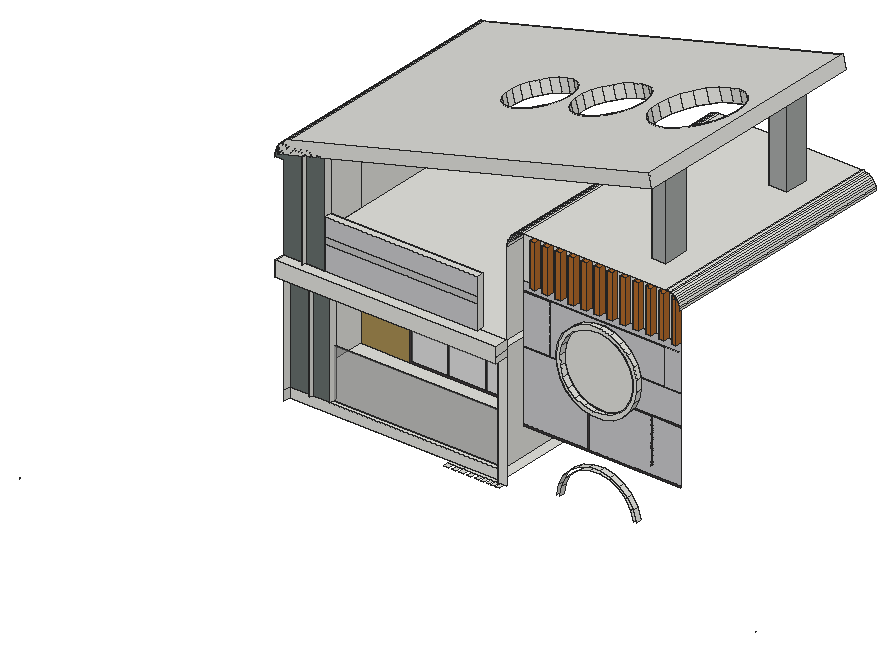
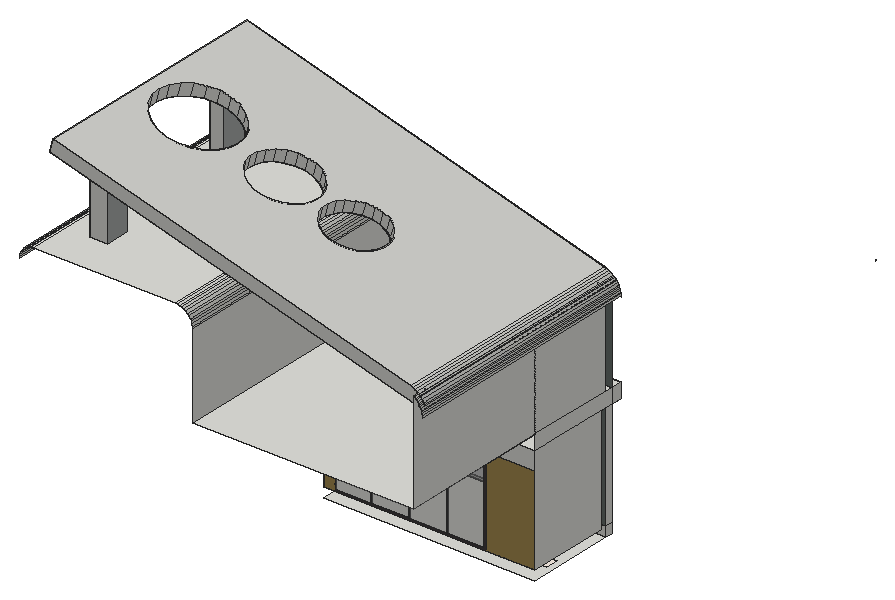
# SketchUp Ruby script. Lengths in inches.
U = 1.inch
M = Sketchup.active_model
def pt(a) = Geom::Point3d.new(a.map { |v| v * U })
def face(e, loops, mat)
  f = e.add_face(loops[0].map { |a| pt(a) })
  loops[1..].each { |l| e.add_face(l.map { |a| pt(a) }).erase! }
  f.material = f.back_material = mat if mat
  f
end
# faces: each face lists its corners as indices into pts; further lists are holes
def faces(e, pts, list, mat = nil) = list.each { |f| face(e, (f[0].is_a?(Array) ? f : [f]).map { |l| l.map { |i| pts[i] } }, mat) }
# xy, xz, yz: faces in a plane at the given z, y or x. An outline is a flat list of corners, or four numbers for a rectangle; further outlines are holes
def ring(l) = l.size == 4 ? [[l[0], l[1]], [l[2], l[1]], [l[2], l[3]], [l[0], l[3]]] : l.each_slice(2).to_a
def flat(e, list, mat, &to3) = list.each { |f| face(e, (f[0].is_a?(Array) ? f : [f]).map { |l| ring(l).map { |u, v| to3.(u, v) } }, mat) }
def xy(e, z, list, mat = nil) = flat(e, list, mat) { |x, y| [x, y, z] }
def xz(e, y, list, mat = nil) = flat(e, list, mat) { |x, z| [x, y, z] }
def yz(e, x, list, mat = nil) = flat(e, list, mat) { |y, z| [x, y, z] }
def lines(e, pts, list) = list.each { |a, b| e.add_line(pt(pts[a]), pt(pts[b])) }
# prism: a flat outline (further loops are holes) pulled along v
def prism(e, loops, v, mat = nil)
  f = face(e, loops, mat); d = Geom::Vector3d.new(v.map { |x| x * U })
  f.pushpull(f.normal.samedirection?(d) ? d.length : -d.length)
end
def box(e, o, s, mat = nil) = prism(e, [[o, [o[0] + s[0], o[1], o[2]], [o[0] + s[0], o[1] + s[1], o[2]], [o[0], o[1] + s[1], o[2]]]], [0, 0, s[2]], mat)
def at(x, y, z, deg = 0) = Geom::Transformation.translation(pt([x, y, z])) * Geom::Transformation.rotation(ORIGIN, Z_AXIS, deg.degrees)
def axes(o, x, y, z) = Geom::Transformation.new([*x, 0, *y, 0, *z, 0, *pt(o).to_a, 1])
def part(name) = M.definitions.add(name)
# library, detail: a bought-in or finely detailed component or shape, given as its bounding box
def library(name, o, s) = part(name).tap { |d| box(d.entities, o, s) }
def detail(e, o, s) = box(e.add_group.entities, o, s)
def put(e, d, t, mat = nil) = e.add_instance(d, t).tap { |i| i.material = mat if mat }
def group(e, t, mat = nil) = e.add_group.tap { |g| g.transformation = t; g.material = mat if mat }.entities
root = M.entities
M.materials.add("Polis06_194").color = [79, 50, 36]
M.materials.add("[0009_Linen]").color = [250, 240, 230]
M.materials.add("[0045_Goldenrod]").color = [218, 165, 32]
M.materials.add("[Asphalt New]").color = [67, 60, 62]
M.materials.add("[Brick Rough Tan]").color = [167, 141, 82]
M.materials.add("[Concrete Form 4x8]").color = [167, 170, 168]
M.materials.add("[Metal Corrugated Shiny]").color = [193, 193, 193]
M.materials.add("[Polished Concrete New]").color = [200, 200, 203]
M.materials.add("[Slate]").color = [102, 110, 108]
M.materials.add("[Translucent Glass Gray]").color = [128, 128, 128]
M.materials["[Translucent Glass Gray]"].alpha = 0.5
M.materials.add("[Wood Bamboo]").color = [177, 105, 43]
c1 = library("Vaso decorativo com seixos\#1",[6.14,-4.72,0],[9.45,4.72,3.26])
c2 = part("群组\#3")
xy(c2.entities,0,[[0,0,4.72,1.18],[0,34.25,4.72,35.43]],"Polis06_194")
xy(c2.entities,85.26,[[0,1.18,4.72,34.25]],"Polis06_194")
xy(c2.entities,86.61,[[0,0,4.72,35.43]],"Polis06_194")
xz(c2.entities,0,[[0,0,4.72,86.61]],"Polis06_194")
xz(c2.entities,1.18,[[0,0,2.36,85.26],[2.36,0,4.72,85.26]],"Polis06_194")
xz(c2.entities,34.25,[[0,0,4.72,85.26]],"Polis06_194")
xz(c2.entities,35.43,[[0,0,4.72,86.61]],"Polis06_194")
yz(c2.entities,0,[[0,0,1.18,86.61],[34.25,0,35.43,86.61],[1.18,85.26,34.25,86.61]],"Polis06_194")
yz(c2.entities,2.36,[[1.18,0,34.25,0,34.25,85.21,1.18,85.26]],"Polis06_194")
yz(c2.entities,4.72,[[0,0,1.18,86.61],[34.25,0,35.43,86.61],[1.18,85.26,34.25,86.61]],"Polis06_194")
xy(root,25308.0625,[[41914.25,35829.26,42429.61,36436.82],[42781.34,35829.26,43218.625,36436.82],[43484.85,35829.26,43975.34,36436.82],[44363.15,35829.26,44725.28,36436.82],[45185.32,35829.26,45537.5,36436.82],
  [45797.6,35829.26,46078.9,36436.82],[46362.66,35829.26,46652.53,36436.82],[46862.23,35829.26,47214.9,36436.82],[47390.11,35829.26,47723.54,36436.82],[41914.25,36436.82,47071.94,36851.76],
  [25070.75,36851.76,47071.94,46071.33]])
xy(root,25456.33,[[25598.07,42633.68,26902.95,43938.55]],"[0009_Linen]")
xy(root,26331.5625,[[27255.29,36569.45,27430.61,36851.76],[29282.19,36851.76,47071.94,37215.15],[29282.19,37327.67,47071.94,37327.67,47071.94,46071.33,25070.75,46071.33,25070.75,37578.54,29282.19,37578.54]])
xy(root,31526.6875,[[29282.19,37215.15,47071.94,37327.67]])
xy(root,37403.375,[[25070.75,34935.13,25070.75,36851.76,27255.29,36851.76,27255.29,36569.45,27430.61,36569.45,27430.61,36851.76,29282.19,36851.76,29282.19,37578.54,25070.75,37578.54,25070.75,46071.33,47071.94,46071.33,47071.94,34935.13],[47071.94,34935.13,48032.1875,36436.82],[27255.29,36569.45,27255.29,36851.76,25070.75,36851.76,25070.75,37578.54,29282.19,37578.54,29282.19,36851.76,27430.61,36851.76,27430.61,36569.45]])
xy(root,38958,[[25070.75,34935.13,48032.1875,34935.13,48032.1875,36436.82,45222.69,36413.97,45222.69,36109.95,27319.9,36109.95,27319.9,35724.07,27192.85,35724.07,27192.85,36109.95,25070.75,36109.95],[27192.85,35724.07,27319.9,35724.07,27319.9,36109.95,29282.19,36109.95,29282.19,36169.9,25070.75,36109.95,27192.85,36109.95],[25070.75,36109.95,29282.19,36169.9,29282.19,36963.36,25070.75,36963.36],[45222.69,36413.97,48032.1875,36436.82,48032.1875,61909.82,25070.75,61909.82,25070.75,36963.36,29282.19,36963.36,29282.19,36839.26,45222.69,36839.26]])
xy(root,44012.3125,[[29282.19,36109.95,45222.69,36839.26]])
xy(root,44199.5625,[[49936.84,36957.88,50535.75,37569.95],[51279.53,36957.88,51878.44,37569.95],[52622.21,36957.88,53221.13,37569.95],[53964.9,36957.88,54563.82,37569.95],[55307.59,36957.88,55906.5,37569.95],
  [56650.28,36957.88,57249.19,37569.95],[57992.96,36957.88,58591.88,37569.95],[59335.65,36957.88,59934.57,37569.95],[60678.34,36957.88,61277.25,37569.95],[62021.03,36957.88,62619.94,37569.95],
  [63363.71,36957.88,63962.63,37569.95],[64706.4,36957.88,65211.19,37569.95]],"[Wood Bamboo]")
xy(root,48641.27,[[65183.27,36436.82,65196.11,36957.88,65211.19,36957.88,65211.19,36436.82],[65196.11,36957.88,65211.19,37569.95,65211.19,36957.88]])
xy(root,48641.27,[[49936.84,36957.88,50535.75,37569.95],[51279.53,36957.88,51878.44,37569.95],[52622.21,36957.88,53221.13,37569.95],[53964.9,36957.88,54563.82,37569.95],[55307.59,36957.88,55906.5,37569.95],
  [56650.28,36957.88,57249.19,37569.95],[57992.96,36957.88,58591.88,37569.95],[59335.65,36957.88,59934.57,37569.95],[60678.34,36957.88,61277.25,37569.95],[62021.03,36957.88,62619.94,37569.95],
  [63363.71,36957.88,63962.63,37569.95],[64706.4,36957.88,65196.11,36957.88,65211.19,37569.95,64706.4,37569.95]],"[Wood Bamboo]")
xy(root,49006.35,[[27192.85,35724.07,27319.9,36109.95]])
xy(root,49453.6875,[[24916.0625,36109.95,25070.75,61909.82],[25070.75,36109.95,29282.19,36963.36],[[49822.99,36436.82,64549.34,61909.82],[60243.78,55175.76,62155.53,57678.95],[60431.21,39788.27,61824.71,42423.59]]])
xy(root,58093.8125,[[60431.21,39788.27,61824.71,42423.59]])
xy(root,58313.875,[[60243.78,55175.76,62155.53,57678.95]])
xz(root,34935.13,[[25070.75,37403.375,48032.1875,38958]])
xz(root,35724.07,[[27192.85,38958,27319.9,49006.35]],"[0045_Goldenrod]")
xz(root,36109.95,[[29282.19,41485.16,45222.69,42077.04]],"[Metal Corrugated Shiny]")
xz(root,36109.95,[[29282.19,38958,45222.69,41485.16],[29282.19,42077.04,45222.69,44012.3125]],"[Polished Concrete New]")
xz(root,36109.95,[[25070.75,38958,27192.85,38958,27192.85,49006.35,27319.9,49006.35,27319.9,38958,29282.19,38958,29282.19,49453.6875,24916.0625,49453.6875,24802.83,49347.6,24696.56,49234.55,24597.67,49114.98,24506.56,48989.39,24423.59,48858.27,24349.11,48722.15,24283.4,48581.59,24226.75,48437.14,24179.36,48289.39,24141.44,48138.93,24113.14,47986.375,24094.5625,47832.33,25070.75,47832.33]],"[Slate]")
xz(root,36436.82,[[47071.94,25308.0625,48032.1875,37403.375]])
xz(root,36569.45,[[27255.29,26331.5625,27430.61,37403.375]],"[0045_Goldenrod]")
xz(root,36839.26,[[29282.19,38958,45222.69,44012.3125]])
xz(root,36851.76,[[25070.75,25308.0625,47071.94,26331.5625]])
xz(root,36851.76,[[25070.75,26331.5625,27255.29,37403.375],[27430.61,26331.5625,29282.19,37403.375]],"[Slate]")
xz(root,36957.88,[[49936.84,44199.5625,50535.75,48641.27],[51279.53,44199.5625,51878.44,48641.27],[52622.21,44199.5625,53221.13,48641.27],[53964.9,44199.5625,54563.82,48641.27],[55307.59,44199.5625,55906.5,48641.27],
  [56650.28,44199.5625,57249.19,48641.27],[57992.96,44199.5625,58591.88,48641.27],[59335.65,44199.5625,59934.57,48641.27],[60678.34,44199.5625,61277.25,48641.27],[62021.03,44199.5625,62619.94,48641.27],
  [63363.71,44199.5625,63962.63,48641.27],[64706.4,44199.5625,65211.19,48641.27]],"[Wood Bamboo]")
xz(root,36963.36,[[25070.75,38958,29282.19,49453.6875]])
xz(root,36996.38,[[[56489.97,34557.29,57592.81,34599.94,58647.03,34926.58,59580.79,35514.94,60330.45,36324.93,60844.93,37301.35,61089.16,38377.65,61046.5,39480.49,60719.86,40534.71,60131.5,41468.47,59321.51,42218.13,58345.1,42732.61,57268.8,42976.84,56165.96,42934.1875,55111.74,42607.55,54177.98,42019.1875,53428.32,41209.2,52913.84,40232.78,52669.6,39156.48,52712.26,38053.64,53038.9,36999.42,53627.26,36065.66,54437.25,35316,55413.66,34801.52],[56529.12,34980.51,55561.02,35200.1875,54682.76,35662.94,53954.2,36337.24,53424.99,37177.125,53131.19,38125.36,53092.82,39117.33,53312.5,40085.43,53775.26,40963.69,54449.56,41692.24,55289.44,42221.46,56237.68,42515.26,57229.65,42553.625,58197.75,42333.94,59076,41871.1875,59804.56,41196.89,60333.77,40357,60627.57,39408.77,60665.94,38416.8,60446.26,37448.7,59983.5,36570.45,59309.21,35841.89,58469.32,35312.68,57521.08,35018.875]]])
xz(root,37327.67,[[29282.19,26331.5625,47071.94,31526.6875]],"[Translucent Glass Gray]")
xz(root,37569.95,[[[56489.97,34557.29,57592.81,34599.94,58647.03,34926.58,59580.79,35514.94,60330.45,36324.93,60330.45,36425.5625,60383.47,36425.5625,60844.93,37301.35,61089.16,38377.65,61046.5,39480.49,60719.86,40534.71,60131.5,41468.47,59321.51,42218.13,58345.1,42732.61,57268.8,42976.84,56165.96,42934.1875,55111.74,42607.55,54177.98,42019.1875,53428.32,41209.2,52913.84,40232.78,52669.6,39156.48,52708.5,38150.94,52712.26,38150.94,52712.26,38053.64,53038.9,36999.42,53627.26,36065.66,54437.25,35316,55413.66,34801.52],[56529.12,34980.51,55561.02,35200.1875,54682.76,35662.94,53954.2,36337.24,53424.99,37177.125,53131.19,38125.36,53092.82,39117.33,53312.5,40085.43,53775.26,40963.69,54449.56,41692.24,55289.44,42221.46,56237.68,42515.26,57229.65,42553.625,58197.75,42333.94,59076,41871.1875,59804.56,41196.89,60333.77,40357,60627.57,39408.77,60665.94,38416.8,60446.26,37448.7,59983.5,36570.45,59309.21,35841.89,58469.32,35312.68,57521.08,35018.875]],[56529.12,34980.51,57521.08,35018.875,58469.32,35312.68,59309.21,35841.89,59983.5,36570.45,60446.26,37448.7,60665.94,38416.8,60627.57,39408.77,60333.77,40357,59804.56,41196.89,59076,41871.1875,58197.75,42333.94,57229.65,42553.625,56237.68,42515.26,55289.44,42221.46,54449.56,41692.24,53775.26,40963.69,53312.5,40085.43,53092.82,39117.33,53131.19,38125.36,53424.99,37177.125,53954.2,36337.24,54682.76,35662.94,55561.02,35200.1875],[60330.45,36324.93,60383.47,36425.5625,60330.45,36425.5625],[52712.26,38053.64,52712.26,38150.94,52708.5,38150.94],[48844.61,44199.5625,49936.84,48641.27],
  [50535.75,44199.5625,51279.53,48641.27],[51878.44,44199.5625,52622.21,48641.27],[53221.13,44199.5625,53964.9,48641.27],[54563.82,44199.5625,55307.59,48641.27],[55906.5,44199.5625,56650.28,48641.27],
  [57249.19,44199.5625,57992.96,48641.27],[58591.88,44199.5625,59335.65,48641.27],[59934.57,44199.5625,60678.34,48641.27],[61277.25,44199.5625,62021.03,48641.27],[62619.94,44199.5625,63363.71,48641.27],
  [63962.63,44199.5625,64706.4,48641.27]])
xz(root,37569.95,[[48844.61,30695.54,65211.19,30888.96],[55508.57,30888.96,55639.38,34661.52],[62132.52,31678.75,62272.21,36324.93],[60330.45,36324.93,62132.52,36324.93,62132.52,36425.5625,60383.47,36425.5625],[62132.52,36324.93,62272.21,36425.5625],
  [62272.21,36324.93,65211.19,36425.5625],[48844.61,38053.64,52712.26,38053.64,52708.5,38150.94,48844.61,38150.94],[51548.6,38150.94,51627.98,43230.47],[61046.5,39480.49,65211.19,39544.76],[63435.76,39544.76,63576.58,43230.47],
  [48844.61,43230.47,63435.76,43362.1],[63435.76,43230.47,63576.58,43362.1],[63576.58,43230.47,65119.73,43362.1]],"[Asphalt New]")
xz(root,37569.95,[[48844.61,30888.96,55508.57,30888.96,55508.57,34661.52,55639.38,34661.52,55639.38,30888.96,65211.19,30888.96,65211.19,36324.93,62272.21,36324.93,62272.21,31678.75,62132.52,31678.75,62132.52,36324.93,60330.45,36324.93,59580.79,35514.94,58647.03,34926.58,57592.81,34599.94,56489.97,34557.29,55413.66,34801.52,54437.25,35316,53627.26,36065.66,53038.9,36999.42,52712.26,38053.64,48844.61,38053.64],[60383.47,36425.5625,65211.19,36425.5625,65211.19,39480.49,61046.5,39480.49,61089.16,38377.65,60844.93,37301.35],[48844.61,38150.94,51548.6,43230.47],[51627.98,38150.94,52708.5,38150.94,52669.6,39156.48,52913.84,40232.78,53428.32,41209.2,54177.98,42019.1875,55111.74,42607.55,56165.96,42934.1875,57268.8,42976.84,58345.1,42732.61,59321.51,42218.13,60131.5,41468.47,60719.86,40534.71,61046.5,39480.49,61046.5,39544.76,63435.76,39544.76,63435.76,43230.47,51627.98,43230.47],[63576.58,39544.76,65211.19,39544.76,65211.19,44199.5625,48844.61,44199.5625,48844.61,43362.1,65119.73,43362.1,65119.73,43230.47,63576.58,43230.47]],"[Polished Concrete New]")
xz(root,37578.54,[[25070.75,26331.5625,29282.19,37403.375]])
xz(root,39788.27,[[60431.21,49453.6875,61824.71,58093.8125]],"[Concrete Form 4x8]")
xz(root,42423.59,[[60431.21,49453.6875,61824.71,58093.8125]])
xz(root,46071.33,[[25070.75,35587.1875,47071.94,37403.375]])
xz(root,46071.33,[[[30221.71,26331.5625,45936.02,35587.1875],[30384.53,26494.39,45773.19,35424.36]],[34111.96,26494.39,34231.7,35424.36],[38078.86,26494.39,38257.17,35424.36],[42015.18,26494.39,42163.14,35424.36]],"[Asphalt New]")
xz(root,46071.33,[[25070.75,26331.5625,30221.71,35587.1875],[45936.02,26331.5625,47071.94,35587.1875]],"[Brick Rough Tan]")
xz(root,46071.33,[[30384.53,26494.39,34111.96,35424.36],[34231.7,26494.39,38078.86,35424.36],[38257.17,26494.39,42015.18,35424.36],[42163.14,26494.39,45773.19,35424.36]],"[Translucent Glass Gray]")
xz(root,55175.76,[[60243.78,49453.6875,62155.53,58313.875]],"[Concrete Form 4x8]")
xz(root,57678.95,[[60243.78,49453.6875,62155.53,58313.875]])
yz(root,25070.75,[[36109.95,25308.0625,36851.76,26331.5625],[36109.95,26331.5625,36851.76,37403.375],[37578.54,26331.5625,46071.33,37403.375],[34935.13,37403.375,36109.95,38958],[36109.95,37403.375,46071.33,38958],
  [36963.36,38958,46071.33,49453.6875],[46071.33,38958,61909.82,49453.6875]])
yz(root,27192.85,[[35724.07,38958,36109.95,49006.35]])
yz(root,27255.29,[[36569.45,26331.5625,36851.76,37403.375]])
yz(root,27319.9,[[35724.07,38958,36109.95,49006.35]])
yz(root,27430.61,[[36569.45,26331.5625,36851.76,37403.375]])
yz(root,29282.19,[[36851.76,26331.5625,37215.15,26331.5625,37215.15,31526.6875,37327.67,31526.6875,37327.67,26331.5625,37578.54,26331.5625,37578.54,37403.375,36851.76,37403.375],[36109.95,38958,36169.9,44012.3125],[36839.26,38958,36839.26,44012.3125,36109.95,44012.3125,36109.95,49453.6875,36963.36,49453.6875,36963.36,38958],[36169.9,38958,36839.26,44012.3125]])
yz(root,45222.69,[[36109.95,38958,36839.26,44012.3125]])
yz(root,47071.94,[[36436.82,25308.0625,36851.76,26331.5625],[36436.82,26331.5625,36436.82,37403.375,46071.33,37403.375,46071.33,26331.5625,37327.67,26331.5625,37327.67,31526.6875,37215.15,31526.6875,37215.15,26331.5625]])
yz(root,48032.1875,[[34935.13,37403.375,36436.82,37977.6875],[34935.13,37977.6875,36436.82,38958],[36436.82,38958,61909.82,47662.89]])
yz(root,49936.84,[[36957.88,44199.5625,37569.95,48641.27]],"[Wood Bamboo]")
yz(root,50535.75,[[36957.88,44199.5625,37569.95,48641.27]],"[Wood Bamboo]")
yz(root,51279.53,[[36957.88,44199.5625,37569.95,48641.27]],"[Wood Bamboo]")
yz(root,51878.44,[[36957.88,44199.5625,37569.95,48641.27]],"[Wood Bamboo]")
yz(root,52622.21,[[36957.88,44199.5625,37569.95,48641.27]],"[Wood Bamboo]")
yz(root,53221.13,[[36957.88,44199.5625,37569.95,48641.27]],"[Wood Bamboo]")
yz(root,53964.9,[[36957.88,44199.5625,37569.95,48641.27]],"[Wood Bamboo]")
yz(root,54563.82,[[36957.88,44199.5625,37569.95,48641.27]],"[Wood Bamboo]")
yz(root,55307.59,[[36957.88,44199.5625,37569.95,48641.27]],"[Wood Bamboo]")
yz(root,55906.5,[[36957.88,44199.5625,37569.95,48641.27]],"[Wood Bamboo]")
yz(root,56650.28,[[36957.88,44199.5625,37569.95,48641.27]],"[Wood Bamboo]")
yz(root,57249.19,[[36957.88,44199.5625,37569.95,48641.27]],"[Wood Bamboo]")
yz(root,57992.96,[[36957.88,44199.5625,37569.95,48641.27]],"[Wood Bamboo]")
yz(root,58591.88,[[36957.88,44199.5625,37569.95,48641.27]],"[Wood Bamboo]")
yz(root,59335.65,[[36957.88,44199.5625,37569.95,48641.27]],"[Wood Bamboo]")
yz(root,59934.57,[[36957.88,44199.5625,37569.95,48641.27]],"[Wood Bamboo]")
yz(root,60243.78,[[55175.76,49453.6875,57678.95,58313.875]],"[Concrete Form 4x8]")
yz(root,60431.21,[[39788.27,49453.6875,42423.59,58093.8125]],"[Concrete Form 4x8]")
yz(root,60678.34,[[36957.88,44199.5625,37569.95,48641.27]],"[Wood Bamboo]")
yz(root,61277.25,[[36957.88,44199.5625,37569.95,48641.27]],"[Wood Bamboo]")
yz(root,61824.71,[[39788.27,49453.6875,42423.59,58093.8125]],"[Concrete Form 4x8]")
yz(root,62021.03,[[36957.88,44199.5625,37569.95,48641.27]],"[Wood Bamboo]")
yz(root,62155.53,[[55175.76,49453.6875,57678.95,58313.875]],"[Concrete Form 4x8]")
yz(root,62619.94,[[36957.88,44199.5625,37569.95,48641.27]],"[Wood Bamboo]")
yz(root,63363.71,[[36957.88,44199.5625,37569.95,48641.27]],"[Wood Bamboo]")
yz(root,63962.63,[[36957.88,44199.5625,37569.95,48641.27]],"[Wood Bamboo]")
yz(root,64706.4,[[36957.88,44199.5625,37569.95,48641.27]],"[Wood Bamboo]")
yz(root,65211.19,[[36957.88,44199.5625,37569.95,48641.27]],"[Wood Bamboo]")
p = [[52992.36,37569.95,25870.1875],[53217.87,37569.95,26863.97],[53217.87,37043.95,26863.97],[52992.36,37043.95,25870.1875],[52913.84,37569.95,26976.35],[52669.6,37569.95,25900.04],
  [52669.6,37043.95,25900.04],[52913.84,37043.95,26976.35],[60425.42,37569.95,27142.75],[60727.02,37569.95,26169.35],[60727.02,37043.95,26169.35],[60425.42,37043.95,27142.75],
  [61046.5,37569.95,26224.05],[60719.86,37569.95,27278.27],[60719.86,37043.95,27278.27],[61046.5,37043.95,26224.05],[53692.9,37569.95,27765.53],[53692.9,37043.95,27765.53],
  [53428.32,37569.95,27952.76],[53428.32,37043.95,27952.76],[59882.17,37569.95,28004.92],[59882.17,37043.95,28004.92],[60131.5,37569.95,28212.03],[60131.5,37043.95,28212.03],
  [54385.09,37569.95,28513.41],[54385.09,37043.95,28513.41],[54177.98,37569.95,28762.75],[54177.98,37043.95,28762.75],[59134.28,37569.95,28697.11],[59134.28,37043.95,28697.11],
  [59321.51,37569.95,28961.69],[59321.51,37043.95,28961.69],[55247.26,37569.95,29056.67],[55247.26,37043.95,29056.67],[58232.73,37569.95,29172.14],[58232.73,37043.95,29172.14],
  [55111.74,37569.95,29351.11],[55111.74,37043.95,29351.11],[58345.1,37569.95,29476.17],[58345.1,37043.95,29476.17],[56220.66,37569.95,29358.26],[56220.66,37043.95,29358.26],
  [57238.94,37569.95,29397.65],[57238.94,37043.95,29397.65],[56165.96,37569.95,29677.75],[56165.96,37043.95,29677.75],[57268.8,37569.95,29720.41],[57268.8,37043.95,29720.41],
  [55413.66,37569.95,34801.52],[56489.97,37569.95,34557.29],[56489.97,36996.38,34557.29],[55413.66,36996.38,34801.52],[57592.81,37569.95,34599.94],[57592.81,36996.38,34599.94],
  [58647.03,37569.95,34926.58],[58647.03,36996.38,34926.58],[54437.25,37569.95,35316],[54437.25,36996.38,35316],[59580.79,37569.95,35514.94],[59580.79,36996.38,35514.94],
  [56529.12,37569.95,34980.51],[55561.02,37569.95,35200.1875],[55561.02,36996.38,35200.1875],[56529.12,36996.38,34980.51],[57521.08,37569.95,35018.875],[57521.08,36996.38,35018.875],
  [58469.32,37569.95,35312.68],[58469.32,36996.38,35312.68],[54682.76,37569.95,35662.94],[54682.76,36996.38,35662.94],[59309.21,37569.95,35841.89],[59309.21,36996.38,35841.89],
  [53627.26,37569.95,36065.66],[53627.26,36996.38,36065.66],[60330.45,37569.95,36324.93],[60330.45,36996.38,36324.93],[53954.2,37569.95,36337.24],[53954.2,36996.38,36337.24],
  [59983.5,37569.95,36570.45],[59983.5,36996.38,36570.45],[53038.9,37569.95,36999.42],[53038.9,36996.38,36999.42],[60383.47,37569.95,36425.5625],[60844.93,37569.95,37301.35],
  [60844.93,36996.38,37301.35],[53424.99,37569.95,37177.125],[53424.99,36996.38,37177.125],[60446.26,37569.95,37448.7],[60446.26,36996.38,37448.7],[52712.26,37569.95,38053.64],
  [52712.26,36996.38,38053.64],[53131.19,37569.95,38125.36],[53131.19,36996.38,38125.36],[61089.16,37569.95,38377.65],[61089.16,36996.38,38377.65],[60665.94,37569.95,38416.8],
  [60665.94,36996.38,38416.8],[52708.5,37569.95,38150.94],[52669.6,36996.38,39156.48],[52669.6,37569.95,39156.48],[53092.82,37569.95,39117.33],[53092.82,36996.38,39117.33],
  [61046.5,37569.95,39480.49],[61046.5,36996.38,39480.49],[60627.57,37569.95,39408.77],[60627.57,36996.38,39408.77],[53312.5,37569.95,40085.43],[53312.5,36996.38,40085.43],
  [52913.84,37569.95,40232.78],[52913.84,36996.38,40232.78],[60333.77,37569.95,40357],[60333.77,36996.38,40357],[60719.86,37569.95,40534.71],[60719.86,36996.38,40534.71],
  [53775.26,37569.95,40963.69],[53775.26,36996.38,40963.69],[53428.32,37569.95,41209.2],[53428.32,36996.38,41209.2],[59804.56,37569.95,41196.89],[59804.56,36996.38,41196.89],
  [60131.5,37569.95,41468.47],[60131.5,36996.38,41468.47],[54449.56,37569.95,41692.24],[54449.56,36996.38,41692.24],[59076,37569.95,41871.1875],[59076,36996.38,41871.1875],
  [54177.98,37569.95,42019.1875],[54177.98,36996.38,42019.1875],[59321.51,37569.95,42218.13],[59321.51,36996.38,42218.13],[55289.44,37569.95,42221.46],[55289.44,36996.38,42221.46],
  [58197.75,37569.95,42333.94],[58197.75,36996.38,42333.94],[55111.74,37569.95,42607.55],[55111.74,36996.38,42607.55],[58345.1,37569.95,42732.61],[58345.1,36996.38,42732.61],
  [56237.68,37569.95,42515.26],[56237.68,36996.38,42515.26],[57229.65,37569.95,42553.625],[57229.65,36996.38,42553.625],[56165.96,37569.95,42934.1875],[56165.96,36996.38,42934.1875],
  [57268.8,37569.95,42976.84],[57268.8,36996.38,42976.84],[48032.1875,36436.82,47662.89],[48047.51,36436.82,47896.63],[48047.51,61909.82,47896.63],[48032.1875,61909.82,47662.89],
  [24094.5625,36109.95,47832.33],[24113.14,36109.95,47986.375],[24113.14,61909.82,47986.375],[24094.5625,61909.82,47832.33],[48093.21,36436.82,48126.38],[48093.21,61909.82,48126.38],
  [66011,36436.82,48171.85],[66023.61,36436.82,47979.42],[66023.61,61909.82,47979.42],[66011,61909.82,48171.85],[24141.44,36109.95,48138.93],[24141.44,61909.82,48138.93],
  [48168.5,36436.82,48348.2],[48168.5,61909.82,48348.2],[24179.36,36109.95,48289.39],[24179.36,61909.82,48289.39],[65973.375,36436.82,48360.98],[65973.375,61909.82,48360.98],
  [24226.75,36109.95,48437.14],[24226.75,61909.82,48437.14],[48272.11,36436.82,48558.29],[48272.11,61909.82,48558.29],[65911.39,36436.82,48543.59],[65911.39,61909.82,48543.59],
  [24283.4,36109.95,48581.59],[24283.4,61909.82,48581.59],[65826.09,36436.82,48716.55],[65826.09,61909.82,48716.55],[48402.25,36436.82,48753.06],[48402.25,61909.82,48753.06],
  [24349.11,36109.95,48722.15],[24349.11,61909.82,48722.15],[65718.96,36436.82,48876.9],[65718.96,61909.82,48876.9],[24423.59,36109.95,48858.27],[24423.59,61909.82,48858.27],
  [48556.7,36436.82,48929.17],[48556.7,61909.82,48929.17],[24506.56,36109.95,48989.39],[24506.56,61909.82,48989.39],[65591.81,36436.82,49021.88],[65591.81,61909.82,49021.88],
  [48732.82,36436.82,49083.625],[48732.82,61909.82,49083.625],[24597.67,36109.95,49114.98],[24597.67,61909.82,49114.98],[65446.82,36436.82,49149.03],[65446.82,61909.82,49149.03],
  [48927.59,36436.82,49213.77],[48927.59,61909.82,49213.77],[24696.56,36109.95,49234.55],[24696.56,61909.82,49234.55],[65286.47,36436.82,49256.17],[65286.47,61909.82,49256.17],
  [49137.68,36436.82,49317.37],[49137.68,61909.82,49317.37],[24802.83,36109.95,49347.6],[24802.83,61909.82,49347.6],[65113.52,36436.82,49341.47],[65113.52,61909.82,49341.47],
  [49359.49,36436.82,49392.67],[49359.49,61909.82,49392.67],[64930.91,36436.82,49403.45],[64930.91,61909.82,49403.45],[24916.0625,36109.95,49453.6875],[24916.0625,61909.82,49453.6875],
  [49589.24,36436.82,49438.37],[49589.24,61909.82,49438.37],[64741.77,36436.82,49441.07],[64741.77,61909.82,49441.07],[49822.99,36436.82,49453.6875],[49822.99,61909.82,49453.6875],
  [64549.34,36436.82,49453.6875],[64549.34,61909.82,49453.6875],[48844.61,37569.95,48641.27],[48844.61,36436.82,48641.27],[48032.1875,36436.82,48333.59],[65305.32,37569.95,44199.5625],
  [65305.32,37569.95,48641.27]]
faces(root,p,[[0,1,2,3],[4,5,6,7],[8,9,10,11],[12,13,14,15],[1,16,17,2],[18,4,7,19],[20,8,11,21],[13,22,23,14],
  [16,24,25,17],[26,18,19,27],[28,20,21,29],[22,30,31,23],[24,32,33,25],[34,28,29,35],[36,26,27,37],[30,38,39,31],
  [32,40,41,33],[42,34,35,43],[44,36,37,45],[40,42,43,41],[38,46,47,39],[46,44,45,47],[48,49,50,51],[49,52,53,50],
  [52,54,55,53],[56,48,51,57],[54,58,59,55],[60,61,62,63],[64,60,63,65],[66,64,65,67],[61,68,69,62],[70,66,67,71],
  [72,56,57,73],[58,74,75,59],[68,76,77,69],[78,70,71,79],[80,72,73,81],[82,83,84,75,74],[76,85,86,77],[87,78,79,88],
  [89,80,81,90],[85,91,92,86],[83,93,94,84],[95,87,88,96],[97,89,90,98,99],[91,100,101,92],[93,102,103,94],[104,95,96,105],
  [100,106,107,101],[108,99,98,109],[110,104,105,111],[102,112,113,103],[106,114,115,107],[116,108,109,117],[118,110,111,119],[112,120,121,113],
  [114,122,123,115],[124,118,119,125],[126,116,117,127],[120,128,129,121],[122,130,131,123],[132,124,125,133],[134,126,127,135],[128,136,137,129],
  [130,138,139,131],[140,132,133,141],[138,140,141,139],[142,134,135,143],[136,144,145,137],[144,142,143,145],[146,147,148,149],[150,151,152,153],
  [147,154,155,148],[156,157,158,159],[151,160,161,152],[154,162,163,155],[160,164,165,161],[166,156,159,167],[164,168,169,165],[162,170,171,163],
  [172,166,167,173],[168,174,175,169],[176,172,173,177],[170,178,179,171],[174,180,181,175],[182,176,177,183],[180,184,185,181],[178,186,187,179],
  [184,188,189,185],[190,182,183,191],[186,192,193,187],[188,194,195,189],[196,190,191,197],[192,198,199,193],[194,200,201,195],[202,196,197,203],
  [198,204,205,199],[200,206,207,201],[208,202,203,209],[204,210,211,205],[212,208,209,213],[206,214,215,207],[210,216,217,211],[218,212,213,219],
  [216,220,221,217],[222,218,219,223]])
lines(root,p,[[224,225],[146,226],[227,228]])
put(root,c1,at(88960.49,17672.72,34376.58))
put(root,c2,at(26473.37,0,34429.41))
g1 = group(root,at(24439.98,36109.95,48164.58))
xz(g1,0,[[0,0,38926.05,10430.2,38580.64,11719.3125,1351,1743.66,1113.83,1666.03,886.53,1563.04,671.79,1435.92,472.17,1286.17,290.04,1115.59,127.56,926.18,-13.34,720.22,-130.97,500.14,-132.8,495.6]])
xz(g1,25275.33,[[0,0,-132.8,495.6,-130.97,500.14,-13.34,720.22,127.56,926.18,290.04,1115.59,472.17,1286.17,671.79,1435.92,886.53,1563.04,1113.83,1666.03,1351,1743.66,38580.64,11719.3125,38926.05,10430.2]])
p = [[-132.8,0,495.6],[-132.8,25275.33,495.6],[0,25275.33,0],[0,0,0],[38926.05,0,10430.2],[38926.05,25275.33,10430.2],
  [29652.81,11881.5625,7945.45],[30061.67,10859.66,8055],[30712.07,9982.14,8229.27],[31559.69,9308.79,8456.39],[32546.77,8885.51,8720.88],[33606.04,8741.13,9004.71],
  [34665.3,8885.51,9288.54],[35652.38,9308.79,9553.03],[36500.01,9982.14,9780.15],[37150.41,10859.66,9954.42],[37559.27,11881.5625,10063.98],[37698.73,12978.19,10101.34],
  [37559.27,14074.83,10063.98],[37150.41,15096.73,9954.42],[36500.01,15974.25,9780.15],[35652.38,16647.6,9553.03],[34665.3,17070.88,9288.54],[33606.04,17215.26,9004.71],
  [32546.77,17070.88,8720.88],[31559.69,16647.6,8456.39],[30712.07,15974.25,8229.27],[30061.67,15096.73,8055],[29652.81,14074.83,7945.45],[29513.35,12978.19,7908.08],
  [21924.48,15118.73,5874.65],[21479.47,14337.02,5755.41],[21245.0625,13462.71,5692.6],[21237.22,12555.37,5690.5],[21456.47,11676.85,5749.25],[21887.89,10887.02,5864.84],
  [22502.0625,10239.7,6029.41],[23257.14,9779,6231.73],[24101.66,9536.32,6458.02],[24978.08,9528.2,6692.86],[25826.66,9755.19,6920.23],[26589.58,10201.82,7124.66],
  [27214.85,10837.66,7292.2],[27659.85,11619.37,7411.43],[27894.26,12493.68,7474.24],[27902.11,13401.02,7476.35],[27682.85,14279.53,7417.6],[27251.4375,15069.37,7302],
  [26637.26,15716.69,7137.43],[25882.1875,16177.39,6935.11],[25037.66,16420.07,6708.82],[24161.25,16428.19,6473.99],[23312.66,16201.2,6246.61],[22549.74,15754.57,6042.1875],
  [20005.09,14382.55,5360.35],[19558.1,15088.84,5240.58],[18949.77,15651.29,5077.58],[18221.55,16031.58,4882.45],[17423.07,16203.79,4668.5],[16608.75,16156.18,4450.3],
  [15834.08,15891.99,4242.73],[15151.86,15429.23,4059.93],[14608.57,14799.4375,3914.35],[14241.24,14045.53,3815.93],[14074.9,13218.89,3771.36],[14120.89,12375.84,3783.68],
  [14376.07,11573.84,3852.06],[14823.0625,10867.55,3971.83],[15431.4,10305.09,4134.83],[16159.61,9924.8,4329.96],[16958.09,9752.6,4543.91],[17772.41,9800.21,4762.1],
  [18547.08,10064.4,4969.68],[19229.31,10527.16,5152.48],[19772.6,11156.95,5298.05],[20139.93,11910.86,5396.48],[20306.27,12737.5,5441.05],[20260.28,13580.55,5428.72],
  [-130.97,0,500.14],[-130.97,25275.33,500.14],[-13.34,0,720.22],[-13.34,25275.33,720.22],[127.56,0,926.18],[127.56,25275.33,926.18],
  [290.04,0,1115.59],[290.04,25275.33,1115.59],[472.17,0,1286.17],[472.17,25275.33,1286.17],[671.79,0,1435.92],[671.79,25275.33,1435.92],
  [886.53,0,1563.04],[886.53,25275.33,1563.04],[1113.83,0,1666.03],[1113.83,25275.33,1666.03],[1351,0,1743.66],[1351,25275.33,1743.66],
  [38580.64,25275.33,11719.3125],[38580.64,0,11719.3125],[29716.25,10859.66,9344.11],[29307.39,11881.5625,9234.55],[29167.94,12978.19,9197.1875],[29307.39,14074.83,9234.55],
  [29716.25,15096.73,9344.11],[30366.66,15974.25,9518.38],[31214.28,16647.6,9745.5],[32201.36,17070.88,10009.99],[33260.625,17215.26,10293.82],[34319.89,17070.88,10577.65],
  [35306.97,16647.6,10842.14],[36154.59,15974.25,11069.26],[36805,15096.73,11243.53],[37213.86,14074.83,11353.09],[37353.3125,12978.19,11390.45],[37213.86,11881.5625,11353.09],
  [36805,10859.66,11243.53],[36154.59,9982.14,11069.26],[35306.97,9308.79,10842.14],[34319.89,8885.51,10577.65],[33260.625,8741.13,10293.82],[32201.36,8885.51,10009.99],
  [31214.28,9308.79,9745.5],[30366.66,9982.14,9518.38],[21134.06,14337.02,7044.52],[21579.0625,15118.73,7163.75],[22204.33,15754.57,7331.29],[22967.25,16201.2,7535.72],
  [23815.83,16428.19,7763.1],[24692.25,16420.07,7997.93],[25536.77,16177.39,8224.22],[26291.85,15716.69,8426.54],[26906.02,15069.37,8591.11],[27337.43,14279.53,8706.71],
  [27556.69,13401.02,8765.46],[27548.85,12493.68,8763.35],[27314.43,11619.37,8700.54],[26869.43,10837.66,8581.31],[26244.17,10201.82,8413.77],[25481.24,9755.19,8209.34],
  [24632.66,9528.2,7981.96],[23756.25,9536.32,7747.13],[22911.72,9779,7520.84],[22156.65,10239.7,7318.52],[21542.47,10887.02,7153.95],[21111.06,11676.85,7038.35],
  [20891.8,12555.37,6979.6],[20899.65,13462.71,6981.71],[19212.6875,15088.84,6529.6875],[19659.68,14382.55,6649.46],[19914.86,13580.55,6717.83],[19960.85,12737.5,6730.16],
  [19794.51,11910.86,6685.59],[19427.18,11156.95,6587.16],[18883.89,10527.16,6441.59],[18201.67,10064.4,6258.78],[17427,9800.21,6051.21],[16612.68,9752.6,5833.02],
  [15814.2,9924.8,5619.06],[15085.98,10305.09,5423.9375],[14477.65,10867.55,5260.9375],[14030.66,11573.84,5141.17],[13775.47,12375.84,5072.79],[13729.48,13218.89,5060.47],
  [13895.82,14045.53,5105.04],[14263.15,14799.4375,5203.46],[14806.44,15429.23,5349.04],[15488.67,15891.99,5531.84],[16263.34,16156.18,5739.41],[17077.66,16203.79,5957.61],
  [17876.14,16031.58,6171.56],[18604.35,15651.29,6366.68],[-345.42,0,-467.15],[-331.8125,0,-217.97],[-291.16,0,28.24],[-223.95,0,268.5625]]
faces(g1,p,[[0,1,2,3],[[4,3,2,5],[6,7,8,9,10,11,12,13,14,15,16,17,18,19,20,21,22,23,24,25,26,27,28,29],[30,31,32,33,34,35,36,37,38,39,40,41,42,43,44,45,46,47,48,49,50,51,52,53],[54,55,56,57,58,59,60,61,62,63,64,65,66,67,68,69,70,71,72,73,74,75,76,77]],[0,78,79,1],[78,80,81,79],[80,82,83,81],[82,84,85,83],[84,86,87,85],[86,88,89,87],
  [88,90,91,89],[90,92,93,91],[92,94,95,93],[[96,95,94,97],[98,99,100,101,102,103,104,105,106,107,108,109,110,111,112,113,114,115,116,117,118,119,120,121],[122,123,124,125,126,127,128,129,130,131,132,133,134,135,136,137,138,139,140,141,142,143,144,145],[146,147,148,149,150,151,152,153,154,155,156,157,158,159,160,161,162,163,164,165,166,167,168,169]],[161,160,65,64],[162,161,64,63],[160,159,66,65],[163,162,63,62],
  [159,158,67,66],[164,163,62,61],[158,157,68,67],[165,164,61,60],[157,156,69,68],[166,165,60,59],[156,155,70,69],[167,166,59,58],
  [155,154,71,70],[168,167,58,57],[154,153,72,71],[169,168,57,56],[153,152,73,72],[146,169,56,55],[152,151,74,73],[147,146,55,54],
  [151,150,75,74],[148,147,54,77],[150,149,76,75],[149,148,77,76],[144,143,34,33],[145,144,33,32],[122,145,32,31],[143,142,35,34],
  [123,122,31,30],[142,141,36,35],[124,123,30,53],[141,140,37,36],[125,124,53,52],[140,139,38,37],[126,125,52,51],[139,138,39,38],
  [127,126,51,50],[138,137,40,39],[128,127,50,49],[137,136,41,40],[129,128,49,48],[136,135,42,41],[130,129,48,47],[135,134,43,42],
  [131,130,47,46],[134,133,44,43],[132,131,46,45],[133,132,45,44],[100,99,6,29],[101,100,29,28],[99,98,7,6],[102,101,28,27],
  [98,121,8,7],[103,102,27,26],[121,120,9,8],[104,103,26,25],[120,119,10,9],[105,104,25,24],[119,118,11,10],[106,105,24,23],
  [118,117,12,11],[107,106,23,22],[117,116,13,12],[108,107,22,21],[116,115,14,13],[109,108,21,20],[115,114,15,14],[110,109,20,19],
  [114,113,16,15],[111,110,19,18],[113,112,17,16],[112,111,18,17],[4,5,96,97]])
lines(g1,p,[[170,171],[171,172],[172,173],[173,0]])
